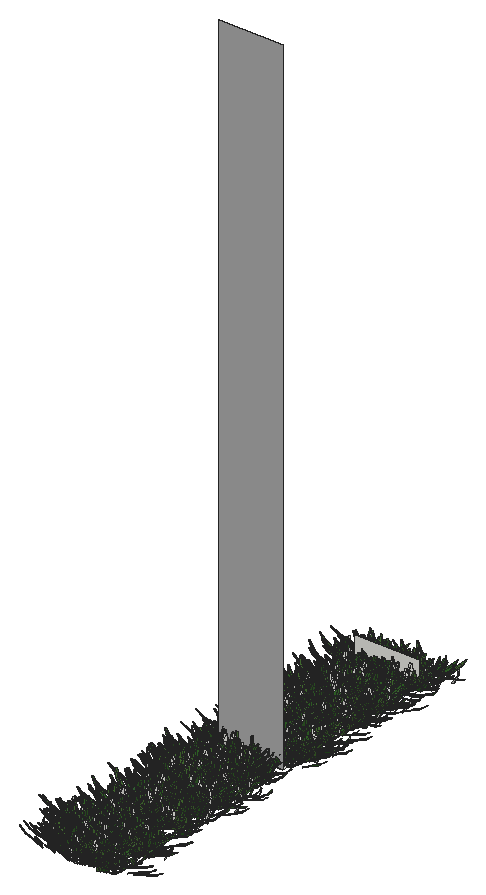
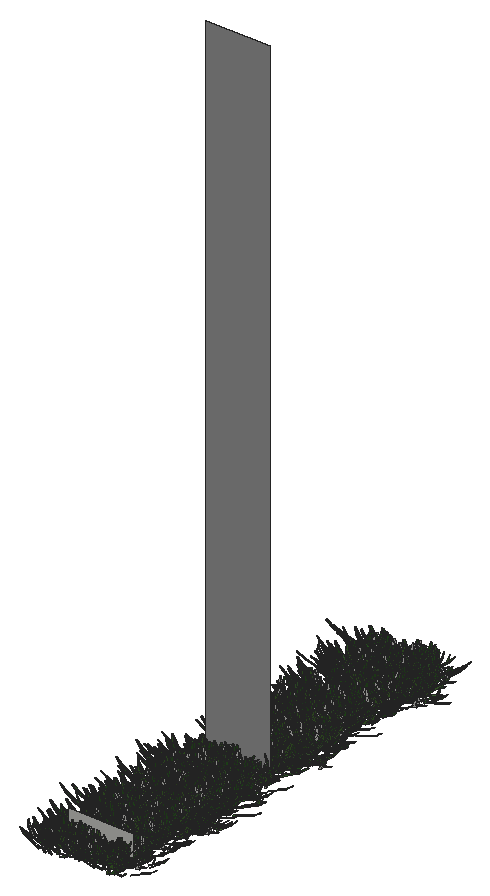
# SketchUp Ruby script. Lengths in inches.
U = 1.inch
M = Sketchup.active_model
def pt(a) = Geom::Point3d.new(a.map { |v| v * U })
def face(e, loops, mat)
  f = e.add_face(loops[0].map { |a| pt(a) })
  loops[1..].each { |l| e.add_face(l.map { |a| pt(a) }).erase! }
  f.material = f.back_material = mat if mat
  f
end
# faces: each face lists its corners as indices into pts; further lists are holes
def faces(e, pts, list, mat = nil) = list.each { |f| face(e, (f[0].is_a?(Array) ? f : [f]).map { |l| l.map { |i| pts[i] } }, mat) }
# xy, xz, yz: faces in a plane at the given z, y or x. An outline is a flat list of corners, or four numbers for a rectangle; further outlines are holes
def ring(l) = l.size == 4 ? [[l[0], l[1]], [l[2], l[1]], [l[2], l[3]], [l[0], l[3]]] : l.each_slice(2).to_a
def flat(e, list, mat, &to3) = list.each { |f| face(e, (f[0].is_a?(Array) ? f : [f]).map { |l| ring(l).map { |u, v| to3.(u, v) } }, mat) }
def xy(e, z, list, mat = nil) = flat(e, list, mat) { |x, y| [x, y, z] }
def xz(e, y, list, mat = nil) = flat(e, list, mat) { |x, z| [x, y, z] }
def yz(e, x, list, mat = nil) = flat(e, list, mat) { |y, z| [x, y, z] }
def lines(e, pts, list) = list.each { |a, b| e.add_line(pt(pts[a]), pt(pts[b])) }
# prism: a flat outline (further loops are holes) pulled along v
def prism(e, loops, v, mat = nil)
  f = face(e, loops, mat); d = Geom::Vector3d.new(v.map { |x| x * U })
  f.pushpull(f.normal.samedirection?(d) ? d.length : -d.length)
end
def box(e, o, s, mat = nil) = prism(e, [[o, [o[0] + s[0], o[1], o[2]], [o[0] + s[0], o[1] + s[1], o[2]], [o[0], o[1] + s[1], o[2]]]], [0, 0, s[2]], mat)
def at(x, y, z, deg = 0) = Geom::Transformation.translation(pt([x, y, z])) * Geom::Transformation.rotation(ORIGIN, Z_AXIS, deg.degrees)
def axes(o, x, y, z) = Geom::Transformation.new([*x, 0, *y, 0, *z, 0, *pt(o).to_a, 1])
def part(name) = M.definitions.add(name)
# library, detail: a bought-in or finely detailed component or shape, given as its bounding box
def library(name, o, s) = part(name).tap { |d| box(d.entities, o, s) }
def detail(e, o, s) = box(e.add_group.entities, o, s)
def put(e, d, t, mat = nil) = e.add_instance(d, t).tap { |i| i.material = mat if mat }
def group(e, t, mat = nil) = e.add_group.tap { |g| g.transformation = t; g.material = mat if mat }.entities
root = M.entities
M.materials.add("Material82").color = [68, 110, 58]
M.materials.add("Material83").color = [48, 90, 38]
M.materials.add("Material84").color = [68, 110, 48]
M.materials.add("Material85").color = [48, 90, 48]
M.materials.add("Material86").color = [58, 110, 58]
M.materials.add("Material87").color = [58, 90, 38]
M.materials.add("Material88").color = [68, 100, 58]
M.materials.add("Material89").color = [48, 100, 38]
M.materials.add("[Color M03]1").color = [170, 170, 170]
c1 = part("grass00")
p = [[-0.6875,0.15,0],[-0.56,0.08,5.52],[-0.04,0.03,2.76],[0.48,-0.02,0],[0.35,-0.02,5.52],[-0.1,-0.14,5.52],
  [-0.12,0.65,8.37],[-0.42,0.65,8.37]]
faces(c1.entities,p,[[0,1,2,3],[3,2,4],[1,5,2],[5,4,2],[1,6,5],[4,5,6],[7,6,1]])
c2 = part("Group16\#1")
put(c2.entities,c1,axes([1.44,-0.61,-0.01],[0.05352,0.12609,0],[-0.10704,0.04543,0.07239],[0.06664,-0.02828,0.11628]),"Material85")
put(c2.entities,c1,axes([0.76,-0.15,-0.01],[0.04676,0.24062,0],[-0.23162,0.04501,0.06642],[0.0652,-0.01267,0.23595]),"Material82")
put(c2.entities,c1,axes([0.79,0.01,-0.01],[-0.00606,0.34651,0],[-0.34381,-0.00602,0.0432],[0.04319,0.00076,0.34386]))
put(c2.entities,c1,axes([1,0.23,-0.01],[-0.07192,0.31144,0],[-0.28722,-0.06632,0.1236],[0.12043,0.02781,0.29478]),"Material84")
put(c2.entities,c1,axes([1.66,0.77,-0.01],[-0.13828,0.29651,0],[-0.21551,-0.1005,0.22471],[0.20365,0.09498,0.23779]),"Material89")
put(c2.entities,c1,axes([0.6875,0.52,-0.01],[-0.18126,0.24051,0],[-0.22746,-0.17142,0.09788],[0.07817,0.05891,0.28481]),"Material84")
put(c2.entities,c1,axes([0.68,0.78,-0.01],[-0.215,0.18688,0],[-0.12385,-0.14248,0.21334],[0.13995,0.16101,0.18878]),"Material82")
put(c2.entities,c1,axes([0.56,1,-0.01],[-0.13756,0.07624,0],[-0.06159,-0.11112,0.0927],[0.04494,0.08108,0.12705]),"Material84")
put(c2.entities,c1,axes([0.2,0.64,-0.01],[-0.23729,0.07254,0],[-0.05711,-0.18681,0.153],[0.04473,0.14632,0.19535]),"Material89")
put(c2.entities,c1,axes([0.0625,0.72,-0.01],[-0.28874,0.02525,0],[-0.02179,-0.24916,0.14647],[0.01276,0.14591,0.25012]),"Material82")
put(c2.entities,c1,axes([-0.08,0.62,-0.01],[-0.34089,-0.04187,0],[0.03255,-0.26504,0.216],[-0.02633,0.21439,0.26703]),"Material89")
put(c2.entities,c1,axes([-0.34,0.98,-0.01],[-0.14314,-0.0493,0],[0.04397,-0.12769,0.06843],[-0.02228,0.0647,0.13505]),"Material89")
put(c2.entities,c1,axes([-0.87,1.45,-0.01],[-0.23488,-0.14114,0],[0.13761,-0.22901,0.06087],[-0.03135,0.05217,0.26717]))
put(c2.entities,c1,axes([-0.72,0.77,-0.01],[-0.14208,-0.13251,0],[0.07209,-0.0773,0.16301],[-0.11118,0.11922,0.1057]),"Material89")
put(c2.entities,c1,axes([-0.62,0.43,-0.01],[-0.14845,-0.21203,0],[0.18654,-0.13061,0.12304],[-0.10079,0.07057,0.22772]),"Material82")
put(c2.entities,c1,axes([-0.68,0.29,-0.01],[-0.13639,-0.32136,0],[0.31723,-0.13464,0.05579],[-0.05136,0.0218,0.34462]),"Material83")
put(c2.entities,c1,axes([-0.64,0.125,-0.01],[-0.0458,-0.23569,0],[0.22124,-0.043,0.08276],[-0.08124,0.01579,0.22538]),"Material86")
put(c2.entities,c1,axes([-1.6,-0.03,-0.01],[0.00576,-0.32897,0],[0.27526,0.00482,0.18018],[-0.18015,-0.00315,0.2753]),"Material84")
put(c2.entities,c1,axes([-1.36,-0.31,-0.01],[0.05718,-0.24765,0],[0.18172,0.04196,0.17267],[-0.16825,-0.03885,0.1865]),"Material89")
put(c2.entities,c1,axes([-1.54,-0.72,-0.01],[0.06537,-0.14017,0],[0.13555,0.06321,0.03939],[-0.0357,-0.01665,0.14956]))
put(c2.entities,c1,axes([-1.19,-0.9,-0.01],[0.09597,-0.12735,0],[0.11214,0.08451,0.07557],[-0.06035,-0.04548,0.14042]),"Material88")
put(c2.entities,c1,axes([-0.47,-0.54,-0.01],[0.11588,-0.10072,0],[0.0618,0.0711,0.12124],[-0.07953,-0.0915,0.0942]))
put(c2.entities,c1,axes([-0.47,-0.84,-0.01],[0.11927,-0.0661,0],[0.06603,0.11913,0.00646],[-0.00313,-0.00565,0.13621]),"Material84")
put(c2.entities,c1,axes([-0.38,-1.24,-0.01],[0.28037,-0.08571,0],[0.0618,0.20215,0.20315],[-0.05939,-0.19428,0.21139]),"Material88")
put(c2.entities,c1,axes([-0.06,-0.66,-0.01],[0.22719,-0.01987,0],[0.01247,0.14255,0.17758],[-0.01547,-0.17691,0.1431]),"Material87")
put(c2.entities,c1,axes([0.11,-0.89,-0.01],[0.14882,0.01828,0],[-0.01058,0.08611,0.12229],[0.01491,-0.12138,0.08676]),"Material85")
put(c2.entities,c1,axes([0.25,-0.72,-0.01],[0.20481,0.07053,0],[-0.06206,0.18022,0.10291],[0.03351,-0.0973,0.1906]),"Material85")
put(c2.entities,c1,axes([0.85,-1.42,-0.01],[0.16481,0.09904,0],[-0.09472,0.15762,0.05616],[0.02893,-0.04814,0.18389]),"Material84")
put(c2.entities,c1,axes([1.01,-1.09,-0.01],[0.21858,0.20385,0],[-0.17495,0.1876,0.15339],[0.10462,-0.11218,0.25652]),"Material89")
put(c2.entities,c1,axes([1.01,-0.71,-0.01],[0.08733,0.12473,0],[-0.06445,0.04512,0.13037],[0.1068,-0.07477,0.07867]),"Material85")
c3 = part("Group15\#1")
put(c3.entities,c2,at(0,0,0))
c4 = part("3darcstudiotree_grass00\#1")
put(c4.entities,c3,at(0,0,0))
xy(root,-29.74,[[1657.0625,1000.12,1674.65,1046.93]])
xz(root,1000.12,[[1657.0625,-29.74,1674.65,149.375]],"[Color M03]1")
xz(root,1046.93,[[1657.0625,-29.74,1674.65,-23.22]])
put(root,c4,axes([1656.66,1026.73,-29.74],[3.58704,0.55594,0],[-1.39662,1.40151,-0.02634],[-0.05335,0.05353,1.58474]))
put(root,c4,axes([1657.29,1011.3,-29.74],[3.13564,-0.95157,0],[2.13614,1.09478,-0.03629],[0.11919,0.06109,1.41389]))
put(root,c4,axes([1656.89,989.93,-29.74],[2.62983,0.98737,0],[-2.70679,1.12128,-0.04733],[-0.14621,0.06057,1.31836]))
put(root,c4,axes([1657.25,952.45,-29.74],[2.45025,1.521,0],[-3.17244,0.79485,-0.05376],[-0.27331,0.06848,1.69687]))
put(root,c4,axes([1657.41,1047.4,-29.74],[3.43516,0.20919,0],[-0.57575,1.47043,-0.03647],[-0.03089,0.0789,1.56991]))
put(root,c4,axes([1657.32,955.45,-29.74],[3.99404,0.60234,0],[-1.558,1.60676,-0.01506],[-0.02517,0.02596,1.52965]))
put(root,c4,axes([1659.16,1028.93,-29.74],[-3.8239,-0.32025,0],[0.87863,-1.63166,-0.02543],[0.02678,-0.04974,1.60712]))
put(root,c4,axes([1659.17,948.67,-29.74],[-3.18903,-1.00454,0],[2.15912,-1.06605,-0.04095],[0.17363,-0.08573,1.76156]))
put(root,c4,axes([1659.25,950.5,-29.74],[1.91072,-1.36379,0],[2.93743,0.64007,-0.00396],[0.02678,0.00583,1.94458]))
put(root,c4,axes([1659.33,953.64,-29.74],[-3.96013,0.90558,0],[-1.84066,-1.25189,-0.01457],[-0.03554,-0.02417,1.33777]))
put(root,c4,axes([1659.96,1023.41,-29.74],[-1.37854,-1.47975,0],[3.2131,-0.46555,-0.02344],[0.115,-0.01666,1.34096]))
put(root,c4,axes([1659.8,1052.93,-29.74],[-3.78694,0.18795,0],[-0.43899,-1.37568,-0.01354],[-0.00909,-0.02849,1.41676]))
put(root,c4,axes([1659.74,1005.67,-29.74],[-3.58928,0.33039,0],[-0.75882,-1.28211,-0.0198],[-0.02657,-0.04489,1.47686]))
put(root,c4,axes([1659.57,1025.13,-29.74],[1.03001,-1.55898,0],[3.46185,0.35573,-0.04641],[0.24674,0.02535,1.47323]))
put(root,c4,axes([1660.32,1020.6,-29.74],[0.07037,-1.71405,0],[4.70144,0.03002,-0.02796],[0.12644,0.00081,1.59394]))
put(root,c4,axes([1659.54,981.91,-29.74],[-1.43633,1.59136,0],[-3.83282,-0.53804,-0.05045],[-0.25445,-0.03572,1.63245]))
put(root,c4,axes([1660.98,961.375,-29.74],[-1.0696,-1.4156,0],[4.38412,-0.5152,-0.01047],[0.05162,-0.00607,1.7643]))
put(root,c4,axes([1660.42,1018.05,-29.74],[-4.25189,0.62806,0],[-1.17044,-1.23238,-0.01358],[-0.02814,-0.02963,1.47772]))
put(root,c4,axes([1659.17,983.55,-29.74],[1.80901,1.52238,0],[-3.47581,0.64237,-0.0367],[-0.2302,0.04254,1.99296]))
put(root,c4,axes([1660.79,1016.5,-29.74],[-4.15804,-0.01553,0],[0.04454,-1.85443,-0.04475],[0.00172,-0.0718,1.43393]))
put(root,c4,axes([1660.67,942.41,-29.74],[-3.28831,-0.06152,0],[0.17407,-1.44709,-0.03298],[0.01066,-0.08861,1.87797]))
put(root,c4,axes([1660.82,992.37,-29.74],[-0.39059,-1.54022,0],[4.16557,-0.16429,-0.04439],[0.19629,-0.00774,1.39437]))
put(root,c4,axes([1660.83,965.88,-29.74],[-3.41271,-0.33865,0],[0.85241,-1.336,-0.02412],[0.03639,-0.05703,1.61843]))
put(root,c4,axes([1660.13,1032.22,-29.74],[2.99211,-0.88341,0],[2.54027,1.33816,-0.01707],[0.06311,0.03325,1.96039]))
put(root,c4,axes([1660.98,1014.76,-29.74],[-3.68076,-0.30441,0],[0.87866,-1.65237,-0.00999],[0.00884,-0.01661,1.38276]))
put(root,c4,axes([1659.67,1040.5,-29.74],[3.8777,-0.38352,0],[0.80355,1.2636,-0.03452],[0.06321,0.0994,1.86367]))
put(root,c4,axes([1661.22,972.43,-29.74],[-2.93694,-0.59609,0],[2.12271,-1.62662,-0.00712],[0.01544,-0.01183,1.64666]))
put(root,c4,axes([1660.7,974.29,-29.74],[-3.29904,0.80499,0],[-2.22234,-1.41651,-0.03047],[-0.07031,-0.04481,1.38852]))
put(root,c4,axes([1660.05,990.88,-29.74],[4.14707,-0.51237,0],[1.30496,1.64274,-0.0458],[0.07431,0.09355,1.7756]))
put(root,c4,axes([1660.625,1028.2,-29.74],[-2.36198,1.34531,0],[-2.91809,-0.79683,-0.03104],[-0.17128,-0.04677,1.78553]))
put(root,c4,axes([1659.73,945.82,-29.74],[3.27777,1.34463,0],[-2.52219,0.95624,-0.03508],[-0.15429,0.0585,1.59982]))
put(root,c4,axes([1660.85,943.98,-29.74],[2.26051,-1.27757,0],[3.2134,0.8843,-0.05108],[0.25562,0.07035,1.79238]))
put(root,c4,axes([1660.46,979.21,-29.74],[-1.59446,1.31407,0],[-3.90941,-0.73777,-0.03408],[-0.12847,-0.02424,1.35762]))
put(root,c4,axes([1661.9,976.57,-29.74],[-0.30604,-1.61832,0],[4.50612,-0.13253,-0.02024],[0.10989,-0.00323,1.84439]))
put(root,c4,axes([1661.09,1003.42,-29.74],[2.97125,-1.188,0],[2.63587,1.02532,-0.00165],[0.00768,0.00299,1.81884]))
put(root,c4,axes([1661.07,968.1,-29.74],[3.41243,-1.19241,0],[2.8473,1.26731,-0.01442],[0.05672,0.02524,1.90876]))
put(root,c4,axes([1660.74,963.68,-29.74],[-1.88838,1.28179,0],[-3.89061,-0.89146,-0.00809],[-0.03969,-0.00909,1.91363]))
put(root,c4,axes([1660.37,1037.89,-29.74],[4.11116,0.47333,0],[-1.05643,1.42708,-0.03197],[-0.04362,0.05892,1.37583]))
put(root,c4,axes([1661.33,994.52,-29.74],[2.99246,-1.30733,0],[3.43775,1.22386,-0.0538],[0.15792,0.05622,1.37259]))
put(root,c4,axes([1662.25,1049.36,-29.74],[-3.25297,-0.61029,0],[1.91072,-1.58399,-0.03826],[0.09019,-0.07477,1.82966]))
put(root,c4,axes([1662.13,998.96,-29.74],[-1.66901,-1.67644,0],[3.86369,-0.59826,-0.05278],[0.29329,-0.04541,1.85719]))
put(root,c4,axes([1662.25,1000.48,-29.74],[-4.35861,-0.14504,0],[0.36663,-1.71363,-0.02802],[0.01298,-0.06068,1.8014]))
put(root,c4,axes([1661.15,958.125,-29.74],[3.20139,-0.30461,0],[0.92111,1.5056,-0.01591],[0.01676,0.0274,1.32206]))
put(root,c4,axes([1660.94,1011.73,-29.74],[3.6615,0.00284,0],[-0.00662,1.32579,-0.0306],[-0.00046,0.09111,1.9022]))
put(root,c4,axes([1662.47,987.83,-29.74],[0.73171,-1.70112,0],[4.49029,0.30039,-0.00997],[0.04273,0.00286,1.48373]))
put(root,c4,axes([1662.36,1010.35,-29.74],[-3.40532,-0.07402,0],[0.22612,-1.61806,-0.00601],[0.00193,-0.01379,1.79325]))
put(root,c4,axes([1662.4375,1044.17,-29.74],[1.09339,-1.57965,0],[4.13626,0.44528,-0.00598],[0.02433,0.00262,1.35627]))
put(root,c4,axes([1661.85,959.29,-29.74],[-2.68631,1.22242,0],[-2.89186,-0.98838,-0.03703],[-0.15503,-0.05299,1.58908]))
put(root,c4,axes([1661.72,1043.42,-29.74],[3.3382,-1.0215,0],[2.0281,1.0308,-0.00126],[0.00417,0.00212,1.3431]))
put(root,c4,axes([1661.08,985.51,-29.74],[1.0764,1.4346,0],[-4.21811,0.49224,-0.04809],[-0.1912,0.02231,1.36712]))
put(root,c4,axes([1661.21,954.95,-29.74],[4.09217,0.10074,0],[-0.26997,1.70555,-0.00965],[-0.00291,0.01837,1.57035]))
put(root,c4,axes([1662.08,1050.76,-29.74],[2.39,-1.25303,0],[3.55352,1.05416,-0.05537],[0.20037,0.05944,1.50911]))
put(root,c4,axes([1661.55,1046.71,-29.74],[3.59653,-0.21085,0],[0.631,1.67397,-0.00967],[0.00626,0.01661,1.41667]))
put(root,c4,axes([1661.35,997.02,-29.74],[1.32449,1.52251,0],[-4.11933,0.55735,-0.02597],[-0.14801,0.02003,1.96681]))
put(root,c4,axes([1661.35,1008.23,-29.74],[3.15923,1.14894,0],[-3.00225,1.28393,-0.03053],[-0.12215,0.05224,1.95907]))
put(root,c4,axes([1662.47,1036.36,-29.74],[-2.42169,0.94143,0],[-3.12641,-1.2508,-0.05994],[-0.19111,-0.07646,1.51606]))
put(root,c4,axes([1661.63,1034.16,-29.74],[1.86247,1.54763,0],[-3.42195,0.64048,-0.01135],[-0.06523,0.01221,1.80626]))
put(root,c4,axes([1662.65,971.02,-29.74],[3.3532,-0.49547,0],[1.21799,1.28203,-0.02122],[0.05381,0.05664,1.88089]))
put(root,c4,axes([1664.63,983.625,-29.74],[-3.17181,-0.36437,0],[1.29907,-1.75875,-0.03129],[0.04635,-0.06275,1.8441]))
put(root,c4,axes([1664.84,1034.68,-29.74],[-3.98386,-0.59662,0],[1.47731,-1.53422,-0.04397],[0.0965,-0.10022,1.92843]))
put(root,c4,axes([1664.8,970.22,-29.74],[-3.51166,-0.15133,0],[0.49376,-1.78204,-0.01667],[0.00952,-0.03434,1.79039]))
put(root,c4,axes([1664.39,1000.95,-29.74],[3.82244,-0.70635,0],[1.81239,1.52539,-0.00986],[0.01787,0.01504,1.36783]))
put(root,c4,axes([1665.25,959.89,-29.74],[-4.25679,0.36903,0],[-0.81289,-1.45836,-0.01858],[-0.01888,-0.03387,1.34303]))
put(root,c4,axes([1665.71,946.42,-29.74],[-2.72023,-1.01034,0],[2.91962,-1.22258,-0.03536],[0.13675,-0.05727,1.8008]))
put(root,c4,axes([1664.85,1049.5,-29.74],[2.33818,-1.41789,0],[2.84176,0.72884,-0.04791],[0.27889,0.07153,1.76421]))
put(root,c4,axes([1665.07,996.96,-29.74],[-2.05483,1.19866,0],[-3.00093,-0.80011,-0.04556],[-0.27207,-0.07254,1.95702]))
put(root,c4,axes([1664.62,1035.5,-29.74],[3.87274,-0.73751,0],[1.55178,1.26734,-0.04306],[0.13654,0.11151,1.95064]))
put(root,c4,axes([1665.35,1018.34,-29.74],[-3.50881,1.16011,0],[-2.69176,-1.26622,-0.04843],[-0.14054,-0.06611,1.41858]))
put(root,c4,axes([1664.68,964.89,-29.74],[-0.97742,1.77445,0],[-3.78925,-0.32463,-0.03052],[-0.14263,-0.01222,1.38983]))
put(root,c4,axes([1664.65,974.65,-29.74],[-0.8481,1.42544,0],[-3.97449,-0.36778,-0.03302],[-0.15824,-0.01464,1.5061]))
put(root,c4,axes([1664.74,1012.76,-29.74],[3.5983,-0.42057,0],[0.96573,1.28508,-0.03127],[0.05191,0.06908,1.48816]))
put(root,c4,axes([1664.74,1010.2,-29.74],[-1.39865,1.66077,0],[-3.78259,-0.49545,-0.00679],[-0.0282,-0.00369,1.30662]))
put(root,c4,axes([1665.54,1023.18,-29.74],[2.65926,-1.384,0],[3.07673,0.91944,-0.04967],[0.23773,0.07104,1.73743]))
put(root,c4,axes([1664.91,1040.71,-29.74],[3.19951,0.37191,0],[-1.24549,1.66647,-0.04213],[-0.05146,0.06886,1.42653]))
put(root,c4,axes([1664.93,1005.14,-29.74],[3.23293,0.85538,0],[-2.19162,1.28829,-0.0468],[-0.14196,0.08345,1.60535]))
put(root,c4,axes([1666,945.21,-29.74],[1.73893,-1.7168,0],[3.5493,0.55914,-0.05078],[0.28442,0.04481,1.72798]))
put(root,c4,axes([1665.2,942.34,-29.74],[1.27117,1.29221,0],[-3.51403,0.53763,-0.02781],[-0.14445,0.0221,1.57422]))
put(root,c4,axes([1666.68,969.07,-29.74],[1.49045,-1.29572,0],[4.01852,0.71892,-0.00454],[0.01627,0.00291,1.30224]))
put(root,c4,axes([1665.45,952.95,-29.74],[3.40006,0.04588,0],[-0.15479,1.78412,-0.02332],[-0.00425,0.049,1.80921]))
put(root,c4,axes([1665.22,988.76,-29.74],[1.48796,1.33204,0],[-3.50735,0.60935,-0.02705],[-0.13278,0.02307,1.54111]))
put(root,c4,axes([1665.64,1038.26,-29.74],[0.11998,1.39847,0],[-4.49149,0.05993,-0.06181],[-0.32467,0.00433,1.77032]))
put(root,c4,axes([1666.66,1032.12,-29.74],[0.37423,-1.77165,0],[3.6892,0.1212,-0.04948],[0.31334,0.01029,1.76318]))
put(root,c4,axes([1666.05,1029.67,-29.74],[-1.23102,1.43236,0],[-4.00109,-0.53481,-0.05878],[-0.24424,-0.03265,1.38915]))
put(root,c4,axes([1667.32,1027.7,-29.74],[-3.85586,-0.61181,0],[1.38378,-1.3564,-0.02256],[0.04705,-0.04612,1.55256]))
put(root,c4,axes([1665.84,1024.7,-29.74],[4.58666,-0.29954,0],[0.76961,1.83286,-0.06031],[0.05541,0.13196,1.9859]))
put(root,c4,axes([1665.59,1044.86,-29.74],[3.04278,1.18912,0],[-3.29647,1.31191,-0.05903],[-0.21773,0.08665,1.83956]))
put(root,c4,axes([1666.92,991.75,-29.74],[-3.4737,0.48099,0],[-1.22806,-1.37939,-0.01418],[-0.03068,-0.03446,1.8149]))
put(root,c4,axes([1665.55,1015.74,-29.74],[2.59618,1.43862,0],[-2.87173,0.80602,-0.01154],[-0.04691,0.01317,1.31865]))
put(root,c4,axes([1667.08,1003.42,-29.74],[0.50435,-1.60129,0],[3.80498,0.18639,-0.05019],[0.26525,0.01299,1.53052]))
put(root,c4,axes([1665.69,981.16,-29.74],[1.0762,1.29593,0],[-3.71861,0.48029,-0.00037],[-0.00166,0.00021,1.37352]))
put(root,c4,axes([1666.51,1050.99,-29.74],[-1.73323,1.28831,0],[-3.70175,-0.77456,-0.05129],[-0.19346,-0.04048,1.34106]))
put(root,c4,axes([1667.4,962.09,-29.74],[-4.57816,0.34958,0],[-0.88534,-1.8033,-0.01839],[-0.0151,-0.03075,1.50803]))
put(root,c4,axes([1667.63,950.24,-29.74],[-1.62742,-1.17488,0],[3.69115,-0.79521,-0.05959],[0.21649,-0.04664,1.30502]))
put(root,c4,axes([1666.85,979.36,-29.74],[1.77469,-1.16148,0],[2.86416,0.68064,-0.04784],[0.28474,0.06767,1.7418]))
put(root,c4,axes([1667.76,985.53,-29.74],[-0.38907,-1.30448,0],[3.64191,-0.16894,-0.01277],[0.06378,-0.00296,1.38207]))
put(root,c4,axes([1666.31,977.57,-29.74],[0.22262,1.70783,0],[-4.21483,0.08545,-0.0387],[-0.20922,0.00424,1.71236]))
put(root,c4,axes([1666.14,966.03,-29.74],[1.40686,1.47706,0],[-4.38712,0.6499,-0.05425],[-0.24934,0.03694,1.72469]))
put(root,c4,axes([1666.5625,995.02,-29.74],[3.74197,-0.40965,0],[1.02528,1.45661,-0.05393],[0.09104,0.12934,1.81331]))
put(root,c4,axes([1666.37,1021.39,-29.74],[3.24935,0.42764,0],[-1.43334,1.69386,-0.04175],[-0.05922,0.06999,1.52086]))
put(root,c4,axes([1668.24,1046.97,-29.74],[-3.23469,-1.08731,0],[2.23739,-1.03522,-0.02002],[0.06548,-0.0303,1.30322]))
put(root,c4,axes([1666.74,1007.24,-29.74],[4.09406,-0.23131,0],[0.47213,1.29969,-0.032],[0.03631,0.09996,1.99674]))
put(root,c4,axes([1667.08,948.56,-29.74],[-1.63246,1.63511,0],[-3.4831,-0.54085,-0.00571],[-0.03452,-0.00536,1.8245]))
put(root,c4,axes([1667.29,958.01,-29.74],[-0.95146,1.7451,0],[-3.70497,-0.31417,-0.03186],[-0.21482,-0.01822,1.95913]))
put(root,c4,axes([1667.17,999.34,-29.74],[1.78223,1.25772,0],[-3.10123,0.68348,-0.02391],[-0.11693,0.02577,1.49173]))
put(root,c4,axes([1667.19,1014.125,-29.74],[0.65139,1.7147,0],[-4.45072,0.26296,-0.01905],[-0.08769,0.00518,1.57029]))
put(root,c4,axes([1668.33,990.52,-29.74],[3.26505,-0.4107,0],[1.3901,1.71877,-0.05774],[0.0978,0.12093,1.91123]))
put(root,c4,axes([1667.95,1042.77,-29.74],[4.04452,0.28903,0],[-0.72611,1.58031,-0.0513],[-0.04641,0.10101,1.54883]))
put(root,c4,axes([1668.17,973.51,-29.74],[2.80643,0.90661,0],[-2.10951,1.0156,-0.00694],[-0.02809,0.01352,1.5947]))
put(root,c4,axes([1668.39,956.04,-29.74],[4.57178,0.1006,0],[-0.19659,1.38952,-0.03032],[-0.00983,0.06951,1.54015]))
put(root,c4,axes([1670.08,990.43,-29.74],[-3.18088,-0.40858,0],[1.35408,-1.63957,-0.00123],[0.00227,-0.00275,1.95221]))
put(root,c4,axes([1670.46,1029.98,-29.74],[-3.04991,-1.12114,0],[2.90905,-1.23081,-0.00052],[0.00199,-0.00084,1.79691]))
put(root,c4,axes([1670.91,955.34,-29.74],[-2.17426,-1.31341,0],[3.93463,-1.01304,-0.04707],[0.15585,-0.04013,1.39282]))
put(root,c4,axes([1670.47,1049.56,-29.74],[0.86182,-1.33711,0],[3.4036,0.34119,-0.00558],[0.03445,0.00345,1.6757]))
put(root,c4,axes([1670.39,1042.06,-29.74],[1.86264,-1.28665,0],[3.53883,0.79678,-0.00497],[0.01917,0.00432,1.35772]))
put(root,c4,axes([1670.55,946.54,-29.74],[-3.35474,0.10257,0],[-0.29043,-1.4774,-0.03359],[-0.01806,-0.09187,1.95875]))
put(root,c4,axes([1670.1875,977.25,-29.74],[3.26089,-0.9276,0],[2.41726,1.32164,-0.00659],[0.02436,0.01332,1.95827]))
put(root,c4,axes([1669.98,942.91,-29.74],[3.92346,-0.38379,0],[1.02863,1.63546,-0.04456],[0.04806,0.07641,1.43455]))
put(root,c4,axes([1670.6875,1045.63,-29.74],[2.18615,-1.3842,0],[3.44906,0.84721,-0.04551],[0.21226,0.05214,1.67334]))
put(root,c4,axes([1671.65,972.5,-29.74],[-3.24318,-0.61658,0],[1.47082,-1.20323,-0.00927],[0.0316,-0.02585,1.99366]))
put(root,c4,axes([1670.49,1032.54,-29.74],[2.25035,1.16277,0],[-2.68664,0.80868,-0.04536],[-0.27393,0.08245,1.92466]))
put(root,c4,axes([1672.2,952.86,-29.74],[-0.91872,-1.28532,0],[4.49567,-0.49978,-0.01485],[0.07367,-0.00819,1.80381]))
put(root,c4,axes([1671.49,966.19,-29.74],[0.6017,-1.37989,0],[3.88457,0.26344,-0.05034],[0.29768,0.02019,1.77282]))
put(root,c4,axes([1670.84,944.49,-29.74],[3.93415,-0.89756,0],[1.9948,1.35987,-0.042],[0.11006,0.07503,1.56273]))
put(root,c4,axes([1671.02,994.13,-29.74],[-1.11116,1.30676,0],[-3.31516,-0.43843,-0.03292],[-0.23061,-0.0305,1.93659]))
put(root,c4,axes([1670.79,1051.8,-29.74],[-1.19077,1.57344,0],[-3.27951,-0.38601,-0.00408],[-0.02113,-0.00249,1.38631]))
put(root,c4,axes([1671.9375,1034.52,-29.74],[-0.12471,-1.80139,0],[4.72201,-0.05084,-0.06757],[0.3331,-0.00359,1.74608]))
put(root,c4,axes([1672.11,1027.62,-29.74],[0.23876,-1.55199,0],[4.36064,0.10434,-0.04584],[0.18368,0.0044,1.3146]))
put(root,c4,axes([1672.38,1010.22,-29.74],[-0.00481,-1.55543,0],[4.64446,-0.00224,-0.02113],[0.08601,-0.00004,1.41674]))
put(root,c4,axes([1671.05,1003.14,-29.74],[3.47227,-0.30693,0],[0.74979,1.31925,-0.01015],[0.01336,0.0235,1.54623]))
put(root,c4,axes([1671.01,1005.14,-29.74],[-1.26342,1.38148,0],[-3.54227,-0.50384,-0.00809],[-0.04856,-0.00691,1.80065]))
put(root,c4,axes([1672.59,1053.54,-29.74],[-2.41696,-1.08887,0],[3.39352,-1.17154,-0.03006],[0.11594,-0.04003,1.73276]))
put(root,c4,axes([1671.66,1011.81,-29.74],[2.94151,-0.90679,0],[2.69176,1.35804,-0.00613],[0.02014,0.01016,1.74641]))
put(root,c4,axes([1670.92,1024.44,-29.74],[0.11831,1.37685,0],[-3.50344,0.04682,-0.00216],[-0.01444,0.00019,1.758]))
put(root,c4,axes([1672.37,979.07,-29.74],[-1.52685,-1.32373,0],[3.20025,-0.57411,-0.03768],[0.23061,-0.04137,1.77164]))
put(root,c4,axes([1671.46,984.47,-29.74],[-1.03634,1.43503,0],[-4.07668,-0.45789,-0.05457],[-0.22787,-0.02559,1.37935]))
put(root,c4,axes([1672.28,1047.4,-29.74],[0.26998,-1.38938,0],[4.08981,0.1236,-0.05496],[0.34231,0.01035,1.9204]))
put(root,c4,axes([1672.58,1015.1,-29.74],[-0.73982,-1.44093,0],[3.74487,-0.29904,-0.04711],[0.2431,-0.01941,1.50792]))
put(root,c4,axes([1671.74,1036.5625,-29.74],[3.32502,-0.81851,0],[2.11953,1.33913,-0.03499],[0.11667,0.07371,1.88939]))
put(root,c4,axes([1672.07,1020.44,-29.74],[2.48182,-1.04217,0],[2.75852,1.02169,-0.02466],[0.10108,0.03744,1.59511]))
put(root,c4,axes([1671.9,1007.79,-29.74],[-2.81085,1.01922,0],[-2.91901,-1.25203,-0.0061],[-0.02341,-0.01004,1.83281]))
put(root,c4,axes([1672.71,985.96,-29.74],[-3.57412,-0.0033,0],[0.00935,-1.57631,-0.04252],[0.00057,-0.09613,1.71753]))
